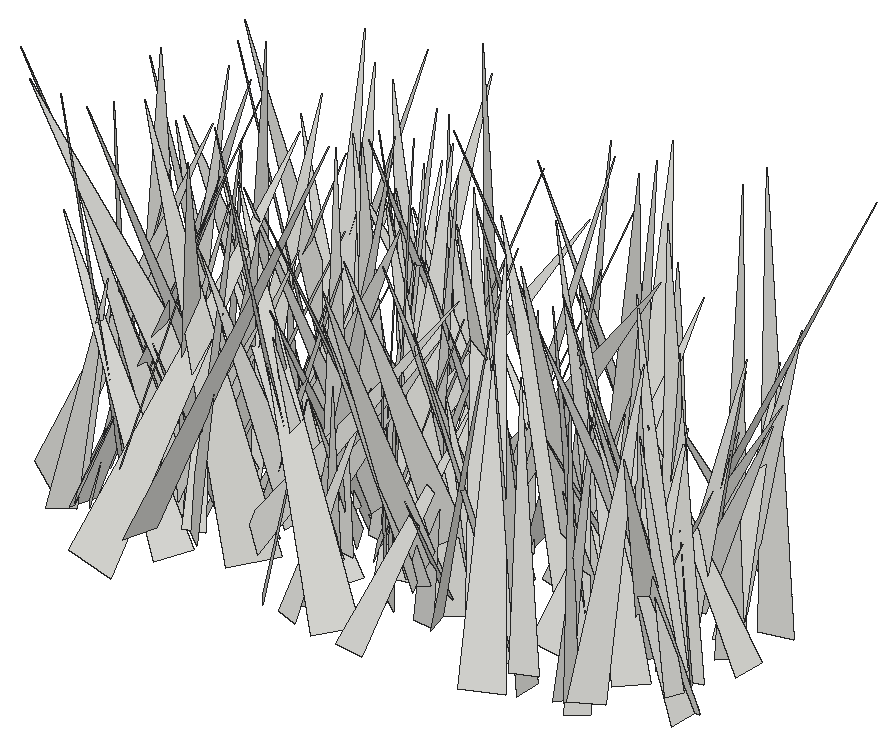
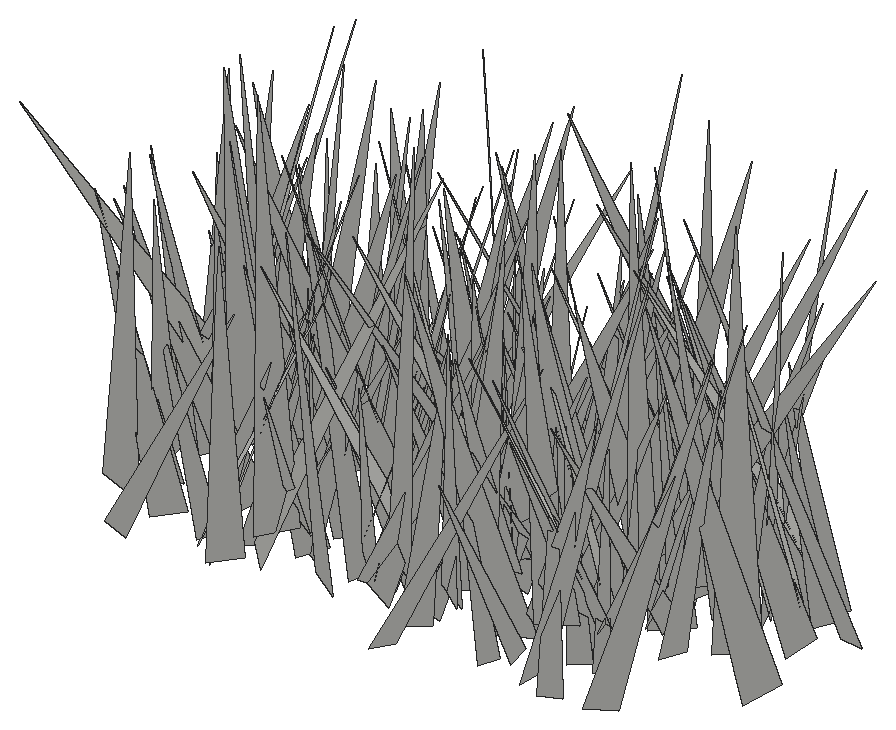
# SketchUp Ruby script. Lengths in inches.
U = 1.inch
M = Sketchup.active_model
def pt(a) = Geom::Point3d.new(a.map { |v| v * U })
def face(e, loops, mat)
  f = e.add_face(loops[0].map { |a| pt(a) })
  loops[1..].each { |l| e.add_face(l.map { |a| pt(a) }).erase! }
  f.material = f.back_material = mat if mat
  f
end
# faces: each face lists its corners as indices into pts; further lists are holes
def faces(e, pts, list, mat = nil) = list.each { |f| face(e, (f[0].is_a?(Array) ? f : [f]).map { |l| l.map { |i| pts[i] } }, mat) }
# xy, xz, yz: faces in a plane at the given z, y or x. An outline is a flat list of corners, or four numbers for a rectangle; further outlines are holes
def ring(l) = l.size == 4 ? [[l[0], l[1]], [l[2], l[1]], [l[2], l[3]], [l[0], l[3]]] : l.each_slice(2).to_a
def flat(e, list, mat, &to3) = list.each { |f| face(e, (f[0].is_a?(Array) ? f : [f]).map { |l| ring(l).map { |u, v| to3.(u, v) } }, mat) }
def xy(e, z, list, mat = nil) = flat(e, list, mat) { |x, y| [x, y, z] }
def xz(e, y, list, mat = nil) = flat(e, list, mat) { |x, z| [x, y, z] }
def yz(e, x, list, mat = nil) = flat(e, list, mat) { |y, z| [x, y, z] }
def lines(e, pts, list) = list.each { |a, b| e.add_line(pt(pts[a]), pt(pts[b])) }
# prism: a flat outline (further loops are holes) pulled along v
def prism(e, loops, v, mat = nil)
  f = face(e, loops, mat); d = Geom::Vector3d.new(v.map { |x| x * U })
  f.pushpull(f.normal.samedirection?(d) ? d.length : -d.length)
end
def box(e, o, s, mat = nil) = prism(e, [[o, [o[0] + s[0], o[1], o[2]], [o[0] + s[0], o[1] + s[1], o[2]], [o[0], o[1] + s[1], o[2]]]], [0, 0, s[2]], mat)
def at(x, y, z, deg = 0) = Geom::Transformation.translation(pt([x, y, z])) * Geom::Transformation.rotation(ORIGIN, Z_AXIS, deg.degrees)
def axes(o, x, y, z) = Geom::Transformation.new([*x, 0, *y, 0, *z, 0, *pt(o).to_a, 1])
def part(name) = M.definitions.add(name)
# library, detail: a bought-in or finely detailed component or shape, given as its bounding box
def library(name, o, s) = part(name).tap { |d| box(d.entities, o, s) }
def detail(e, o, s) = box(e.add_group.entities, o, s)
def put(e, d, t, mat = nil) = e.add_instance(d, t).tap { |i| i.material = mat if mat }
def group(e, t, mat = nil) = e.add_group.tap { |g| g.transformation = t; g.material = mat if mat }.entities
root = M.entities
c1 = part("fur_instance\#9")
p = [[0.8125,0,1.79],[0.67,-0.02,1.48],[0,-0.11,0],[0,0.11,0]]
faces(c1.entities,p,[[0,1,2,3]])
put(root,c1,axes([110.68,143.55,-27.1],[-4.80095,-0.85986,1.55653],[-1.24807,4.82151,-1.18603],[1.26668,1.49164,4.73094]))
put(root,c1,axes([102.17,146.74,-27.1],[1.78326,-6.33726,0.7797],[-6.26284,-1.89367,-1.06754],[-1.24322,0.44943,6.49625]))
put(root,c1,axes([97.64,143.97,-28.22],[-2.4957,-1.61977,2.11338],[-2.18018,2.90599,-0.34732],[1.52869,1.50005,2.95492]))
put(root,c1,axes([90.87,145.6,-28.22],[-5.20637,-5.83633,2.28098],[-6.06397,5.44004,0.07832],[1.57922,1.64775,7.82067]))
put(root,c1,axes([108.52,143.81,-27.1],[-0.93822,4.8343,1.08723],[4.93478,0.81164,0.64956],[-0.44769,-1.18472,4.88147]))
put(root,c1,axes([93.6,144.44,-28.22],[-4.33384,4.15795,0.46311],[4.09626,4.08164,1.68703],[-0.85069,-1.52868,5.76409]))
put(root,c1,axes([88.85,144.6,-28.22],[3.46953,-2.67132,1.40146],[-2.94376,-3.4648,0.68347],[-0.65905,1.41311,4.3251]))
put(root,c1,axes([97.93,145.97,-27.1],[4.25123,5.18566,4.75994],[6.35301,-5.22113,0.01405],[-3.03108,-3.67013,6.70551]))
put(root,c1,axes([93.1,143.33,-27.1],[8.11647,0.24258,0.67526],[0.10402,-7.98511,1.61836],[-0.70993,1.60345,7.95719]))
put(root,c1,axes([98.96,143.56,-28.22],[1.39427,3.92432,0.17719],[3.92808,-1.39069,-0.10895],[0.04345,-0.20342,4.16322]))
put(root,c1,axes([111.26,143.62,-27.1],[-4.2045,3.84796,1.64776],[3.68267,4.51063,-1.13666],[1.98995,-0.21727,5.58504]))
put(root,c1,axes([110.55,143.23,-27.1],[-4.99347,0.21503,1.45697],[-0.36457,4.80955,-1.95935],[1.42691,1.98134,4.59803]))
put(root,c1,axes([100.76,143.81,-28.22],[-3.57557,6.64036,0.56629],[6.42877,3.26724,2.27945],[-1.75672,-1.55901,7.1891]))
put(root,c1,axes([99.07,145.63,-27.1],[-2.91756,2.69263,1.56889],[3.08399,2.80363,0.92331],[0.448,-1.76443,3.86133]))
put(root,c1,axes([102.05,146.43,-27.1],[-4.72142,-2.258,0.83052],[-2.14472,4.77905,0.80066],[1.09019,-0.37724,5.17198]))
put(root,c1,axes([94.5,144.28,-27.1],[4.33311,5.30156,2.10924],[5.44411,-4.63436,0.46433],[-1.70794,-1.32191,6.83131]))
put(root,c1,axes([111.07,147.46,-27.1],[4.81338,-2.70132,0.36004],[-2.51999,-4.69011,-1.49931],[-1.0375,-1.14068,5.31205]))
put(root,c1,axes([106.91,143.66,-28.22],[-2.95766,6.66869,1.17233],[6.76114,2.97762,0.11972],[0.36439,-1.12067,7.29416]))
put(root,c1,axes([92.13,147.43,-27.1],[7.49694,-1.26912,1.50095],[-0.87324,-7.45265,-1.93987],[-1.76095,-1.70734,7.35199]))
put(root,c1,axes([91.85,142.31,-28.22],[0.04279,8.23701,0.26485],[7.98617,0.02394,-2.03491],[2.0346,-0.26721,7.98181]))
put(root,c1,axes([95.89,145.69,-28.22],[-5.61004,5.72169,2.32507],[6.16954,5.3361,1.75473],[0.28367,-2.89906,7.81865]))
put(root,c1,axes([104.23,144.7,-27.1],[4.8135,2.02359,1.54657],[1.94555,-5.05552,0.55956],[-1.64367,-0.05793,5.19149]))
put(root,c1,axes([98.9,145.99,-27.1],[-0.48959,-3.44443,1.08487],[-3.54488,0.6673,0.51889],[0.68909,0.98557,3.44014]))
put(root,c1,axes([103.34,146.375,-27.1],[-4.54236,-5.48641,0.31776],[-5.31376,4.27953,-2.06985],[-1.40202,1.55551,6.81539]))
put(root,c1,axes([88.68,145.33,-28.22],[3.29573,-2.04708,1.27302],[-2.29025,-3.33183,0.57152],[-0.75223,1.17531,3.83742]))
put(root,c1,axes([94.33,144.57,-27.1],[-1.12302,3.48075,0.37457],[3.50037,1.10997,0.18007],[-0.0574,-0.41163,3.65299]))
put(root,c1,axes([106.38,146.09,-28.22],[-5.00716,-3.11226,0.75462],[-3.18598,4.98296,-0.58898],[0.32424,0.90067,5.86608]))
put(root,c1,axes([107.99,144.66,-28.22],[-7.03444,-1.19576,1.59787],[-1.52444,6.99776,-1.47438],[1.28808,1.75153,6.98136]))
put(root,c1,axes([92.9,146.18,-28.22],[-6.42244,0.41118,0.57395],[0.45958,6.42194,0.54196],[0.53597,-0.57954,6.41273]))
put(root,c1,axes([102.97,147.66,-27.1],[2.20766,-6.15742,1.48059],[-5.96151,-2.54967,-1.71445],[-2.13691,0.75174,6.31254]))
put(root,c1,axes([109.11,146.13,-27.1],[3.12486,4.78234,3.10342],[5.39282,-3.6275,0.15986],[-1.8492,-2.49745,5.71052]))
put(root,c1,axes([92.16,144.55,-27.1],[3.27247,4.57721,0.86039],[4.6176,-3.3258,0.13012],[-0.60735,-0.62316,5.62521]))
put(root,c1,axes([101.89,143.08,-28.22],[-3.33289,3.23483,0.32122],[2.5841,2.91556,-2.549],[1.97223,1.64647,3.88264]))
put(root,c1,axes([93.54,147.79,-27.1],[-7.87957,1.88276,1.17896],[2.17634,7.41366,2.70618],[0.44527,-2.91806,7.63603]))
put(root,c1,axes([96.59,147.23,-27.1],[-4.94323,1.53486,1.76986],[2.06825,4.80019,1.61379],[1.10026,-2.12747,4.91803]))
put(root,c1,axes([98.81,147.49,-27.1],[-3.02452,-1.82217,1.01563],[-1.34667,3.07159,1.50047],[1.5932,-0.86291,3.19635]))
put(root,c1,axes([112.83,146.83,-28.22],[-1.48365,-5.76059,1.44193],[-5.8771,1.21156,-1.20691],[-0.85046,1.67706,5.82486]))
put(root,c1,axes([96.05,145.46,-27.1],[4.06376,5.39951,0.02576],[4.83357,-3.62337,-3.0294],[2.40665,-1.8401,6.04083]))
put(root,c1,axes([100.4,146.83,-28.22],[3.47548,2.68418,2.07766],[3.24177,-3.50628,-0.89294],[-1.00618,-2.02524,4.29959]))
put(root,c1,axes([91.62,146.09,-28.22],[2.31497,4.33574,1.17317],[4.28428,-1.73503,-2.04175],[1.34907,-1.93005,4.47091]))
put(root,c1,axes([113.14,146.35,-28.22],[-5.40823,0.65228,0.52882],[0.69912,5.40686,0.48075],[0.46513,-0.5426,5.42617]))
put(root,c1,axes([101.09,146.23,-28.22],[-2.0645,-2.99831,1.70133],[-3.28642,2.31061,0.08412],[1.04107,1.34824,3.63936]))
put(root,c1,axes([110.25,144.41,-28.22],[-4.64664,1.60589,0.29185],[1.45378,4.47236,-1.46283],[0.74202,1.29401,4.69365]))
put(root,c1,axes([95.84,148.3,-27.1],[4.75134,-2.11282,0.36953],[-1.90852,-4.57438,-1.61505],[-0.97883,-1.33672,4.94275]))
put(root,c1,axes([89.14,145.34,-28.22],[6.02676,-0.13267,0.65935],[-0.25057,-5.95995,1.09109],[-0.62414,1.1116,5.92866]))
put(root,c1,axes([108.95,147.74,-28.22],[2.57242,-3.23839,0.522],[-3.12857,-2.6216,-0.84629],[-0.98573,-0.13048,4.04824]))
put(root,c1,axes([102.36,146.3125,-27.1],[0.25275,3.74041,1.98428],[3.79537,-1.08135,1.55493],[-1.87703,-1.68284,3.41127]))
put(root,c1,axes([101.22,146.03,-27.1],[5.9616,4.7587,3.0284],[5.08757,-6.43918,0.10304],[-2.43578,-1.80245,7.62727]))
put(root,c1,axes([90.5,146.03,-28.22],[-6.27895,-2.5321,2.5957],[-2.9165,6.61067,-0.60625],[2.15482,1.56906,6.74309]))
put(root,c1,axes([110.46,149.4375,-28.22],[-6.83559,-3.49227,1.59422],[-2.83471,6.78714,2.71329],[2.5888,-1.7893,7.18049]))
put(root,c1,axes([104.95,146.61,-28.22],[-3.28307,2.60382,1.30489],[2.8552,3.26547,0.66758],[0.57484,-1.34832,4.13676]))
put(root,c1,axes([95.17,147.3,-28.22],[-3.35024,-7.10363,1.41562],[-6.97339,2.74138,-2.74705],[-1.95891,2.39017,7.35795]))
put(root,c1,axes([87.25,145.76,-28.22],[3.97232,6.71602,1.21655],[6.692,-3.55551,-2.22255],[1.34242,-2.14887,7.47961]))
put(root,c1,axes([94.24,146.09,-27.1],[-5.6206,-6.05261,0.8091],[-5.56666,4.62654,-4.06048],[-2.5102,3.29256,7.1929]))
put(root,c1,axes([99.08,146.4,-28.22],[-4.10469,4.34568,0.4298],[4.19686,3.76273,2.03626],[-1.20665,-1.6956,5.62024]))
put(root,c1,axes([92.24,146.1,-28.22],[3.62784,4.7769,0.79864],[4.78599,-3.38301,-1.50576],[0.74217,-1.53438,5.80626]))
put(root,c1,axes([94.74,147.2,-28.22],[5.29628,3.42643,1.15131],[3.61426,-4.98862,-1.7797],[0.0553,-2.11891,6.05175]))
put(root,c1,axes([113.14,145.79,-27.1],[-4.26519,0.30143,0.24037],[0.24291,4.17451,-0.92459],[0.29939,0.9072,4.17466]))
put(root,c1,axes([105.97,145.31,-28.22],[-3.06885,7.2619,1.47031],[7.40414,2.94663,0.90053],[-0.27521,-1.70206,7.83212]))
put(root,c1,axes([92.33,148.63,-28.22],[3.94338,-5.9757,0.15667],[-5.94055,-3.89659,0.90015],[0.66588,0.62564,7.10275]))
put(root,c1,axes([105.65,146.7,-28.22],[-4.03311,-0.04964,1.55556],[-0.10181,4.31995,-0.1261],[1.55302,0.15428,4.03144]))
put(root,c1,axes([111.67,145.41,-27.1],[-1.94953,6.2532,0.70862],[6.08536,1.68405,1.8809],[-1.60411,-1.2111,6.27419]))
put(root,c1,axes([98.69,146.45,-27.1],[1.00735,6.64791,2.58508],[7.07427,-1.26504,0.49655],[-0.91221,-2.46923,6.70544]))
put(root,c1,axes([89.21,145.5625,-28.22],[-3.93965,-2.75758,3.63418],[-3.8658,4.56754,-0.72493],[2.42222,2.80458,4.7539]))
put(root,c1,axes([99,144.63,-28.22],[-7.34355,0.30763,3.29021],[-0.75169,7.65215,-2.39318],[3.21793,2.48952,6.94946]))
put(root,c1,axes([96.85,147.48,-27.1],[3.67258,4.04026,0.63824],[3.75616,-2.99162,-2.6759],[1.61937,-2.22383,4.75932]))
put(root,c1,axes([110.73,149.3,-28.22],[-5.87389,-5.06073,1.31002],[-4.91563,6.01764,1.20596],[1.77871,-0.08191,7.65893]))
put(root,c1,axes([90,143.94,-27.1],[6.02604,4.35688,0.13616],[4.14402,-5.7981,2.12678],[-1.35204,1.64734,7.12547]))
put(root,c1,axes([103.22,149.06,-27.1],[-5.52274,-3.05851,1.02558],[-2.84433,5.57616,1.31266],[1.52186,-0.67738,6.17511]))
put(root,c1,axes([88.31,147.01,-28.22],[6.73911,-0.51973,0.37006],[-0.5475,-6.72675,0.52311],[-0.32757,0.55072,6.73884]))
put(root,c1,axes([99.74,147.16,-27.1],[4.36053,2.62617,0.62372],[2.69593,-4.29581,-0.7602],[-0.13318,-0.97427,5.03319]))
put(root,c1,axes([97.71,147.59,-28.22],[1.13242,-3.28388,1.61058],[-3.44754,-1.52145,-0.67814],[-1.2216,1.24962,3.40681]))
put(root,c1,axes([89.6,146.86,-27.1],[5.1332,2.66859,0.80867],[2.72409,-5.16107,-0.26035],[-0.59552,-0.60587,5.77956]))
put(root,c1,axes([89.5,148.96,-27.1],[2.09335,-3.21544,0.11512],[-3.16402,-2.08217,-0.6229],[-0.58423,-0.24481,3.78592]))
put(root,c1,axes([103.08,146.95,-28.22],[-2.35431,6.5098,1.98677],[6.74258,1.94391,1.62058],[-0.92858,-2.38982,6.73008]))
put(root,c1,axes([98.02,149.58,-28.22],[-1.09873,-5.30096,0.04279],[-5.29764,1.09638,-0.20521],[-0.19227,0.08352,5.40974]))
put(root,c1,axes([93.02,146.5,-28.22],[5.4364,3.24485,0.19999],[3.25087,-5.4295,-0.27539],[-0.03035,-0.33899,6.32516]))
put(root,c1,axes([104.1,148.95,-27.1],[-0.46017,-7.01963,1.64197],[-7.20868,0.46604,-0.02793],[0.07879,1.64032,7.03464]))
put(root,c1,axes([96.26,148.68,-28.22],[0.42808,-6.23217,1.75974],[-6.34467,-0.7568,-1.13683],[-1.29687,1.64535,6.14254]))
put(root,c1,axes([110.33,148.58,-27.1],[-1.30366,-3.70433,0.26528],[-3.50778,1.13584,-1.37745],[-1.21983,0.69265,3.67753]))
put(root,c1,axes([99.96,148.47,-28.22],[-2.1287,-6.56011,1.58213],[-6.38568,1.42177,-2.69649],[-2.18201,2.23898,6.34786]))
put(root,c1,axes([106.7,149.6875,-28.22],[0.47812,-7.3143,1.47747],[-7.45136,-0.54714,-0.29732],[-0.39895,1.45332,7.32388]))
put(root,c1,axes([94.05,149.28,-28.22],[1.4912,-7.63112,1.5604],[-7.07021,-0.65953,3.53123],[3.26816,2.05513,6.92734]))
put(root,c1,axes([102.6875,145.93,-28.22],[3.07038,6.62387,1.59445],[6.28566,-3.42873,2.13997],[-2.62838,-0.46188,6.98022]))
put(root,c1,axes([110.42,147.46,-27.1],[-0.72601,3.76819,0.7458],[3.80081,0.81458,-0.41575],[0.55615,-0.64789,3.8149]))
put(root,c1,axes([112.07,146.99,-27.1],[-0.60049,6.11637,0.8715],[5.86899,0.29123,2.00004],[-1.92986,-1.0175,5.81123]))
put(root,c1,axes([94.93,148.15,-27.1],[4.2362,2.18763,0.04516],[2.18011,-4.21144,-0.49393],[0.18673,-0.4595,4.74206]))
put(root,c1,axes([99.28,149.35,-28.22],[6.19787,3.91116,1.13836],[4.069,-5.84754,-2.06304],[0.19042,-2.34857,7.0324]))
put(root,c1,axes([101.18,148.93,-28.22],[-5.53788,-5.2946,2.37412],[-5.70348,5.57065,-0.88067],[1.06751,2.29618,7.61087]))
put(root,c1,axes([93.05,147.67,-27.1],[-5.05417,-1.27819,2.14403],[-1.86511,5.15169,-1.32541],[1.65892,1.89778,5.04199]))
put(root,c1,axes([90.97,147.55,-28.22],[1.99412,7.08431,1.8343],[7.27705,-2.12036,0.27805],[-0.77249,-1.68678,7.35436]))
put(root,c1,axes([97.76,149.62,-27.1],[6.10585,-2.9623,2.45846],[-2.96929,-6.55789,-0.52733],[-2.45002,0.56525,6.76598]))
put(root,c1,axes([111.49,148.24,-28.22],[-0.81741,7.52572,2.31704],[7.8363,0.54876,0.98214],[-0.77303,-2.39493,7.506]))
put(root,c1,axes([106.72,148.76,-27.1],[-3.37701,5.49526,1.43426],[5.6473,3.0721,1.52623],[-0.60248,-2.00587,6.26679]))
put(root,c1,axes([98.41,149.2,-27.1],[-3.74017,-2.83655,2.38458],[-3.12746,4.23356,0.13062],[1.98777,1.32365,4.69232]))
put(root,c1,axes([98.09,149.83,-27.1],[-0.66847,-3.61729,0.84651],[-3.58891,0.40659,-1.09666],[-0.95975,0.99906,3.51127]))
put(root,c1,axes([100.27,147.73,-28.22],[-2.23719,7.0676,1.63885],[7.20712,2.3619,-0.34736],[0.83319,-1.45336,7.40509]))
put(root,c1,axes([88.46,150.125,-27.1],[5.05478,-5.09898,2.04992],[-5.28407,-5.27475,-0.09077],[-1.51011,1.38923,7.17929]))
put(root,c1,axes([110.14,149.46,-27.1],[-4.58199,0.67037,2.42399],[0.81188,5.16228,0.10702],[2.38033,-0.47034,4.62953]))
put(root,c1,axes([106.97,147.09,-28.22],[-1.51128,6.4389,0.97646],[6.11666,1.74753,-2.05657],[2.23592,-0.42848,6.28601]))
put(root,c1,axes([111.89,148.27,-28.22],[-4.46035,-2.40279,1.6408],[-2.85913,4.17643,-1.65628],[0.53948,2.26814,4.788]))
put(root,c1,axes([92.61,149.76,-27.1],[7.55648,0.00384,2.83421],[0.13477,-8.06186,-0.34839],[-2.831,-0.37353,7.54844]))
put(root,c1,axes([92.86,150.8125,-28.22],[-2.16973,-4.86696,0.63571],[-4.9077,2.16207,-0.19771],[0.07681,0.6613,5.32503]))
put(root,c1,axes([109.23,147.63,-28.22],[-7.36083,-0.13148,0.37404],[-0.23398,7.05478,-2.12469],[0.32007,2.13349,7.04874]))
put(root,c1,axes([107.65,147.88,-28.22],[-2.69846,2.82224,0.09608],[2.72603,2.63813,-0.93001],[0.73688,0.57546,3.79233]))
put(root,c1,axes([112.76,150.11,-28.22],[-4.33776,1.46199,0.55548],[1.55819,4.18055,1.16497],[0.13425,-1.28363,4.42678]))
put(root,c1,axes([103.84,149.875,-27.1],[-3.08604,-1.58363,1.00431],[-1.62158,3.22493,0.10239],[0.94181,0.36349,3.46714]))
put(root,c1,axes([101.96,151.76,-28.22],[-5.41835,-3.58553,1.38238],[-3.2455,5.54933,1.6725],[2.0576,-0.68883,6.27832]))
put(root,c1,axes([94.92,150.2,-27.1],[-1.35927,-4.19334,1.10265],[-4.18909,0.97193,-1.4678],[-1.11869,1.45561,4.1566]))
put(root,c1,axes([110.62,149.34,-27.1],[0.08637,4.97569,1.67082],[5.15736,0.22998,-0.95146],[0.97504,-1.65717,4.88463]))
put(root,c1,axes([104.13,149.55,-28.22],[-3.43885,-1.25141,0.28396],[-1.28081,3.29756,-0.97876],[-0.07859,1.01608,3.52615]))
put(root,c1,axes([108.58,148.81,-27.1],[2.96295,7.07925,2.39249],[7.30087,-3.29107,0.69644],[-1.59283,-1.91622,7.64263]))
put(root,c1,axes([93.59,149.92,-28.22],[3.27603,2.91205,0.73309],[2.99826,-3.11162,-1.03833],[0.1671,-1.26001,4.25844]))
put(root,c1,axes([107.72,149.01,-27.1],[-1.2405,4.10694,0.41743],[4.03089,1.11105,1.04764],[-0.89058,-0.69186,4.16031]))
put(root,c1,axes([92.15,149.8,-27.1],[-6.45817,-1.9042,0.82118],[-2.02073,6.38203,-1.093],[0.4658,1.28531,6.64374]))
put(root,c1,axes([104.35,150.51,-28.22],[0.8957,-3.44027,0.95903],[-3.38159,-0.49886,1.36875],[1.14894,1.21373,3.28089]))
put(root,c1,axes([100.18,148.3,-27.1],[-5.70534,2.42628,0.74712],[2.22137,5.6608,-1.42016],[1.22905,1.03174,6.03498]))
put(root,c1,axes([110.01,150.54,-27.1],[2.80159,-3.67069,0.58517],[-3.61323,-2.51742,1.50747],[0.87232,1.36159,4.36468]))
put(root,c1,axes([99.35,147.8,-27.1],[2.9038,6.51052,1.10748],[6.2299,-3.10193,1.9005],[-2.1913,-0.1914,6.87074]))
put(root,c1,axes([93.42,148.02,-27.1],[-5.22484,3.83291,1.4033],[3.4058,5.3502,-1.93269],[2.24967,0.80218,6.18505]))
put(root,c1,axes([98.45,149.49,-27.1],[-2.02202,5.92033,1.45384],[6.05855,1.78151,1.17164],[-0.67672,-1.74024,6.14542]))
put(root,c1,axes([110.16,150.9,-27.1],[5.07227,1.20948,1.05659],[1.39553,-5.05165,-0.91676],[-0.7948,-1.15114,5.13326]))
put(root,c1,axes([94.71,151.35,-27.1],[-5.73221,-5.07274,1.73381],[-5.23258,5.8463,-0.19467],[1.1657,1.29813,7.652]))
put(root,c1,axes([98.41,150.37,-27.1],[2.1369,3.02619,1.55246],[3.28055,-2.31782,0.00255],[-0.89775,-1.26656,3.70461]))
put(root,c1,axes([104.76,151.89,-28.22],[-3.74984,-6.28849,1.24601],[-6.40364,3.74219,-0.38514],[0.30173,1.26879,7.3115]))
put(root,c1,axes([109.38,148.76,-27.1],[-5.51425,5.90533,1.65371],[5.90522,5.71303,-0.71018],[1.6541,-0.70927,8.04832]))
put(root,c1,axes([99.53,147.88,-27.1],[5.91646,3.40669,0.5347],[3.12979,-5.75065,2.00759],[-1.44773,1.49011,6.52531]))
put(root,c1,axes([106.18,150.65,-28.22],[-4.30239,2.31555,0.00735],[2.25428,4.18495,1.12996],[-0.52922,-0.99839,4.75348]))
put(root,c1,axes([99.84,151.51,-28.22],[4.31656,-7.06636,0.27005],[-6.24466,-3.6606,4.0303],[3.31821,2.3034,7.23345]))
put(root,c1,axes([107.97,150.61,-28.22],[4.90095,-2.69617,0.00541],[-2.57457,-4.67657,1.67032],[0.80058,1.46597,5.33842]))
put(root,c1,axes([87.39,150.17,-28.22],[6.84778,-1.68967,1.39359],[-1.92956,-6.81846,1.21431],[-1.03628,1.53061,6.94784]))
put(root,c1,axes([96.99,147.75,-27.1],[-7.37463,3.18086,0.67882],[2.84062,7.11825,-2.49505],[1.58417,2.04365,7.63399]))
put(root,c1,axes([105.21,150.9,-28.22],[2.79577,3.11606,1.7882],[3.42019,-3.00212,-0.11591],[-1.09992,-1.41467,4.18482]))
put(root,c1,axes([102.04,149.54,-28.22],[3.37937,2.22818,0.23171],[2.15143,-3.34494,0.78826],[-0.62436,0.53406,3.97033]))
put(root,c1,axes([93.55,149.2,-27.1],[0.65103,4.23875,0.31259],[3.78552,-0.72206,1.9071],[-1.9325,0.01355,3.84107]))
put(root,c1,axes([107.45,149.87,-27.1],[-5.34624,-2.21651,3.3319],[-3.00843,5.89263,-0.90721],[2.6389,2.22728,5.71596]))
put(root,c1,axes([100.18,149.1875,-28.22],[-0.0626,5.05917,0.30688],[5.04763,0.09003,-0.45456],[0.45914,-0.29998,5.03909]))
put(root,c1,axes([102.3125,152.125,-28.22],[6.84395,0.46131,0.76105],[0.6015,-6.74756,-1.31919],[-0.65589,-1.3745,6.73144]))
put(root,c1,axes([97.42,149.32,-27.1],[2.23337,6.49328,0.05356],[5.9184,-2.0122,-2.84202],[2.67172,-0.9705,6.25089]))
put(root,c1,axes([102.76,149.27,-27.1],[4.44163,5.80553,0.93246],[5.82565,-4.50337,0.28854],[-0.79717,-0.56325,7.30404]))
put(root,c1,axes([92.73,151.07,-27.1],[4.81991,2.46867,0.79438],[2.57067,-4.76928,-0.77622],[-0.3421,-1.05666,5.35942]))
put(root,c1,axes([99.32,151.62,-28.22],[5.36084,-0.19835,3.29768],[0.06393,-6.27827,-0.48156],[-3.30302,-0.44345,5.34285]))
put(root,c1,axes([93.22,152.28,-28.22],[1.83451,-3.56347,0.05806],[-3.52397,-1.80394,0.62811],[0.53227,0.33851,3.95843]))
put(root,c1,axes([90.01,151.51,-27.1],[-4.92159,1.07561,1.43405],[1.22896,5.07505,0.41117],[1.30503,-0.72281,5.02095]))
put(root,c1,axes([92.21,152.43,-28.22],[-0.97115,-4.17934,0.95629],[-4.09852,1.19278,1.05068],[1.25838,0.65947,4.16006]))
put(root,c1,axes([101.3,152.6875,-28.22],[-2.75065,-6.97463,1.22589],[-6.99898,2.47729,-1.60986],[-1.07823,1.71227,7.32256]))
put(root,c1,axes([99.05,152.72,-28.22],[-0.13278,-3.81265,0.23397],[-3.74221,0.08288,-0.77308],[-0.76609,0.25594,3.73581]))
put(root,c1,axes([109.92,147.83,-27.1],[7.75154,3.11882,0.30174],[2.75499,-7.16733,3.30818],[-1.4927,2.96765,7.67264]))
put(root,c1,axes([104.5,151.93,-28.22],[4.10289,-2.86128,0.97197],[-3.01034,-4.01302,0.89377],[-0.2636,1.29386,4.92156]))
put(root,c1,axes([105.98,152.97,-28.22],[-5.74525,-5.95088,0.61636],[-5.93253,5.55629,-1.65334],[-0.77329,1.58601,8.10478]))
put(root,c1,axes([106.43,152.76,-28.22],[-3.60372,1.36671,1.25031],[1.68423,3.55609,0.96723],[0.77106,-1.37995,3.73084]))
put(root,c1,axes([91.5625,149.82,-27.1],[4.67368,1.9817,0.84614],[1.46066,-4.3994,2.23565],[-1.58416,1.79011,4.55767]))
put(root,c1,axes([92.39,151.68,-27.1],[-3.14834,2.92622,0.07201],[2.87738,3.07451,0.86494],[-0.53726,-0.68166,4.21031]))
put(root,c1,axes([105.02,153.15,-27.1],[6.65936,-3.07974,1.86174],[-3.09449,-6.89952,-0.34452],[-1.83712,0.458,7.32893]))
put(root,c1,axes([101.55,152.32,-28.22],[-3.57331,4.48467,0.98446],[4.4978,3.16833,1.89248],[-0.92266,-1.92337,5.41289]))
put(root,c1,axes([90.84,154.1875,-28.22],[5.01755,-2.86523,2.69296],[-2.1597,-5.65647,-1.99435],[-3.28592,-0.6574,5.42291]))
put(root,c1,axes([108.59,151.87,-28.22],[-1.92431,3.57441,0.40694],[3.46774,1.72017,1.28872],[-0.95749,-0.95373,3.84949]))
put(root,c1,axes([97.7,152.125,-27.1],[-5.4066,3.91291,1.98693],[4.14231,5.59139,0.26032],[1.44915,-1.38406,6.66892]))
put(root,c1,axes([111.07,151.08,-28.22],[-0.62067,4.74172,0.56344],[4.77083,0.63973,-0.12835],[0.20124,-0.5417,4.78044]))
put(root,c1,axes([97.77,150.45,-27.1],[-1.13883,5.42731,0.08742],[5.42427,1.13458,0.2244],[-0.2017,-0.13157,5.54096]))
put(root,c1,axes([102.22,151.79,-28.22],[1.055,3.81063,1.04337],[3.83467,-1.24762,0.6792],[-0.95124,-0.80317,3.89521]))
put(root,c1,axes([100.95,150.47,-28.22],[5.73522,3.47371,0.17785],[3.39582,-5.66618,1.16354],[-0.75282,0.90483,6.60345]))
put(root,c1,axes([100.52,152.44,-27.1],[-3.60643,-6.53276,3.39182],[-7.2869,3.70246,-0.61691],[1.0404,3.28673,7.43658]))
put(root,c1,axes([93.3125,151.16,-28.22],[-0.33332,4.6985,0.41104],[4.65173,0.39553,-0.74898],[0.77866,-0.35159,4.65038]))
put(root,c1,axes([107.81,153.15,-28.22],[3.40491,-1.73217,0.1961],[-1.74293,-3.39081,0.31125],[-0.03288,0.3664,3.80749]))
put(root,c1,axes([107.01,153.86,-28.22],[-6.81995,-3.62088,0.84533],[-3.65528,6.85252,-0.13797],[0.68141,0.51893,7.72033]))
put(root,c1,axes([108.05,153.23,-28.22],[-4.80301,-2.64529,0.12183],[-2.62964,4.73476,-0.865],[-0.31202,0.81591,5.41463]))
put(root,c1,axes([93.86,153.74,-28.22],[-7.83608,-0.63477,1.59162],[-0.4911,7.96997,0.76075],[1.64165,-0.64574,7.82485]))
put(root,c1,axes([92.46,151.8,-27.1],[1.86244,4.7215,0.55373],[4.68693,-1.72429,-1.06173],[0.79484,-0.89561,4.96326]))
put(root,c1,axes([94.17,152.27,-27.1],[-2.76968,5.79414,2.34049],[6.07448,3.09716,-0.47899],[1.46654,-1.88589,6.4042]))
put(root,c1,axes([109.71,152.84,-28.22],[-1.7832,4.7887,2.83203],[5.02838,2.65983,-1.33139],[2.38064,-2.03113,4.93345]))
put(root,c1,axes([111.82,150.3125,-28.22],[-7.67594,0.43258,1.18162],[-0.05572,7.18028,-2.99063],[1.25708,2.9597,7.0826]))
put(root,c1,axes([105.1,151.57,-28.22],[0.25291,3.93977,0.05992],[3.89833,-0.25892,0.57035],[-0.57304,-0.02262,3.90646]))
put(root,c1,axes([110.45,154.67,-28.22],[-0.19761,-4.29399,0.26182],[-4.09062,0.10641,-1.34218],[-1.33181,0.31028,4.08362]))
put(root,c1,axes([92.64,154.54,-28.22],[0.8236,-4.35079,0.44599],[-4.32851,-0.74586,0.71716],[0.62636,0.56649,4.3696]))
put(root,c1,axes([95.25,151.89,-28.22],[-1.50811,5.89701,0.63499],[5.61901,1.21081,2.10069],[-1.89858,-1.1007,5.71281]))
put(root,c1,axes([97.83,153.12,-27.1],[2.36348,3.65871,1.87372],[3.9267,-2.64879,0.21906],[-1.21573,-1.4425,4.3502]))
put(root,c1,axes([98.92,153.625,-28.22],[-4.02078,2.93374,1.78068],[3.22926,4.16274,0.43339],[1.1617,-1.41743,4.95839]))
put(root,c1,axes([95.6,153.98,-28.22],[3.66443,-1.25509,0.51627],[-1.25966,-3.69872,-0.05095],[-0.50503,0.11865,3.87307]))
put(root,c1,axes([95.99,152.15,-28.22],[-1.25446,7.26591,1.58891],[7.27727,1.53186,-1.25954],[1.53602,-1.32352,7.26503]))
put(root,c1,axes([93.53,150.75,-27.1],[4.16098,5.56887,0.17793],[5.30628,-4.02846,1.99315],[-1.69922,1.05685,6.65984]))
put(root,c1,axes([106.39,154.07,-28.22],[4.30224,-3.16543,2.15858],[-3.43037,-4.62804,0.05027],[-1.70646,1.32286,5.34104]))
put(root,c1,axes([98.93,155.3,-28.22],[-5.99784,0.36822,0.31916],[0.44096,5.77868,1.61988],[0.20737,-1.63795,5.78668]))
put(root,c1,axes([112.01,152.41,-28.22],[0.70044,7.59304,1.85976],[7.56257,-1.13109,1.76971],[-1.98005,-1.63401,7.41708]))
put(root,c1,axes([97.98,152.93,-27.1],[1.64216,5.46326,1.64146],[5.44457,-2.0108,1.24565],[-1.70244,-1.16093,5.56707]))
put(root,c1,axes([95.08,153.11,-28.22],[3.56009,0.21869,0.65734],[0.01468,-3.46445,1.07311],[-0.69261,1.05069,3.40155]))
put(root,c1,axes([102.92,153.31,-28.22],[3.25616,5.95918,2.11371],[6.15078,-3.5363,0.49462],[-1.46542,-1.60155,6.77272]))
